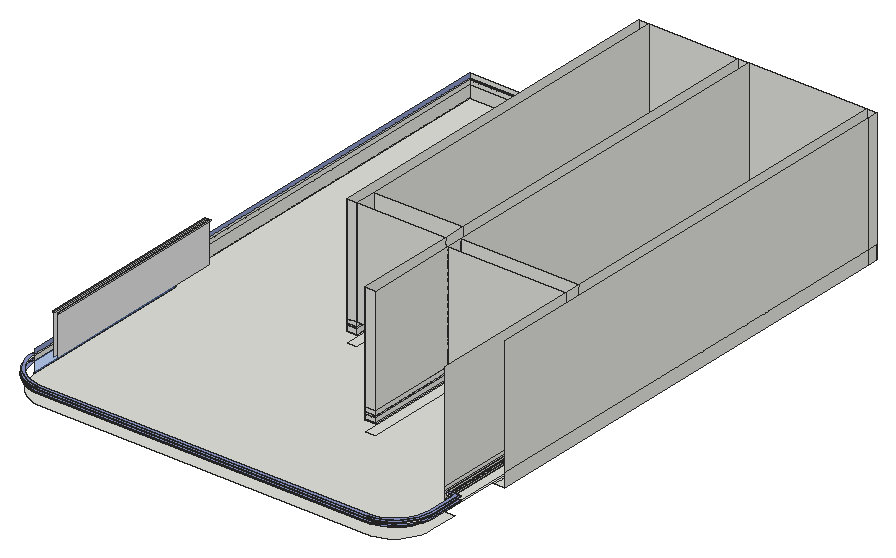
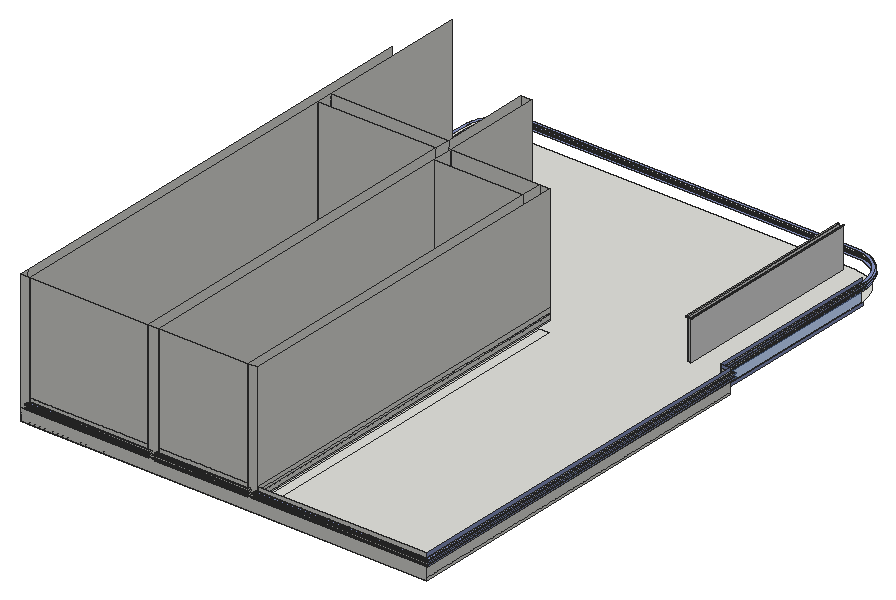
# SketchUp Ruby script. Lengths in inches.
U = 1.inch
M = Sketchup.active_model
def pt(a) = Geom::Point3d.new(a.map { |v| v * U })
def face(e, loops, mat)
  f = e.add_face(loops[0].map { |a| pt(a) })
  loops[1..].each { |l| e.add_face(l.map { |a| pt(a) }).erase! }
  f.material = f.back_material = mat if mat
  f
end
# faces: each face lists its corners as indices into pts; further lists are holes
def faces(e, pts, list, mat = nil) = list.each { |f| face(e, (f[0].is_a?(Array) ? f : [f]).map { |l| l.map { |i| pts[i] } }, mat) }
# xy, xz, yz: faces in a plane at the given z, y or x. An outline is a flat list of corners, or four numbers for a rectangle; further outlines are holes
def ring(l) = l.size == 4 ? [[l[0], l[1]], [l[2], l[1]], [l[2], l[3]], [l[0], l[3]]] : l.each_slice(2).to_a
def flat(e, list, mat, &to3) = list.each { |f| face(e, (f[0].is_a?(Array) ? f : [f]).map { |l| ring(l).map { |u, v| to3.(u, v) } }, mat) }
def xy(e, z, list, mat = nil) = flat(e, list, mat) { |x, y| [x, y, z] }
def xz(e, y, list, mat = nil) = flat(e, list, mat) { |x, z| [x, y, z] }
def yz(e, x, list, mat = nil) = flat(e, list, mat) { |y, z| [x, y, z] }
def lines(e, pts, list) = list.each { |a, b| e.add_line(pt(pts[a]), pt(pts[b])) }
# prism: a flat outline (further loops are holes) pulled along v
def prism(e, loops, v, mat = nil)
  f = face(e, loops, mat); d = Geom::Vector3d.new(v.map { |x| x * U })
  f.pushpull(f.normal.samedirection?(d) ? d.length : -d.length)
end
def box(e, o, s, mat = nil) = prism(e, [[o, [o[0] + s[0], o[1], o[2]], [o[0] + s[0], o[1] + s[1], o[2]], [o[0], o[1] + s[1], o[2]]]], [0, 0, s[2]], mat)
def at(x, y, z, deg = 0) = Geom::Transformation.translation(pt([x, y, z])) * Geom::Transformation.rotation(ORIGIN, Z_AXIS, deg.degrees)
def axes(o, x, y, z) = Geom::Transformation.new([*x, 0, *y, 0, *z, 0, *pt(o).to_a, 1])
def part(name) = M.definitions.add(name)
# library, detail: a bought-in or finely detailed component or shape, given as its bounding box
def library(name, o, s) = part(name).tap { |d| box(d.entities, o, s) }
def detail(e, o, s) = box(e.add_group.entities, o, s)
def put(e, d, t, mat = nil) = e.add_instance(d, t).tap { |i| i.material = mat if mat }
def group(e, t, mat = nil) = e.add_group.tap { |g| g.transformation = t; g.material = mat if mat }.entities
root = M.entities
M.materials.add("0326 AP 7207 CLASSIC PURPLE").color = [140, 152, 201]
M.materials.add("[Color M06]").color = [86, 86, 86]
M.materials.add("[Color M07]").color = [58, 58, 58]
M.materials.add("[Mirror 02]").color = [229, 229, 229]
M.materials.add("[Translucent Glass Blue]").color = [100, 149, 237]
M.materials["[Translucent Glass Blue]"].alpha = 0.5
xy(root,252,[[228.58,142.3125,330.09,142.75],[37.41,142.75,46.41,142.75,46.41,566.25,2.97,566.25,2.97,220.92,10.38,220.92,10.38,221.67,12.4,221.67,12.4,221.45,14.34,221.45,14.34,220.92,37.41,220.92],[46.41,142.75,181.41,557.25],[181.41,142.75,190.41,557.25],[190.41,142.75,364.41,557.25],
  [364.41,142.75,373.41,557.25],[10.38,220.92,11.125,220.92,11.125,221.45,12.4,221.45,12.4,221.67,10.38,221.67],[11.125,220.92,12.4,221.45],[12.4,220.92,14.34,221.45],[46.41,557.25,181.41,566.25],
  [181.41,557.25,190.41,566.25],[190.41,557.25,364.41,566.25],[364.41,557.25,373.41,566.25]])
xy(root,252,[[228.58,138.25,330.09,142.3125]],"[Color M07]")
xy(root,254.0625,[[45.79,26.25,340.59,26.25,344.88,26.53,349.09,27.37,353.15,28.75,357,30.65,360.57,33.03,363.8,35.86,364.41,36.56,366.625,39.09,369.01,42.66,370.91,46.51,372.29,50.57,373.125,54.78,373.41,59.0625,373.41,86.25,364.41,86.25,364.41,566.25,257.02,566.25,257.02,141.25,247.2,141.25,247.2,566.25,166.41,566.25,166.41,233.75,157.41,233.75,157.41,566.25,2.97,566.25,2.97,220.92,11.66,220.92,11.66,60.38,11.95,55.92,12.82,51.55,14.25,47.32,16.23,43.31,18.71,39.6,21.65,36.25,25.01,33.3,28.72,30.82,32.73,28.85,36.95,27.41,41.33,26.54]])
xy(root,264,[[364.41,86.25,373.41,566.25],[247.2,141.25,257.02,566.25],[157.41,233.75,166.41,566.25]])
xy(root,264.4375,[[[45.79,24.43,41.09,24.74,36.48,25.66,32.03,27.17,27.8125,29.25,23.9,31.86,20.37,34.96,17.27,38.5,14.66,42.41,12.58,46.625,11.07,51.08,10.15,55.6875,9.84,60.38,9.84,219.11,1.15,219.11,1.15,568.07,159.22,568.07,159.22,235.56,164.59,235.56,164.59,568.07,249.02,568.07,249.02,143.07,255.2,143.07,255.2,568.07,366.22,568.07,366.22,88.07,375.22,88.07,375.22,59,374.93,54.54,374.05,50.1,372.59,45.81,370.59,41.75,368.07,37.98,365.77,35.36,365.08,34.57,361.68,31.59,357.91,29.07,353.85,27.07,349.56,25.61,345.11,24.73,340.65,24.43],[45.79,26.25,340.59,26.25,344.88,26.53,349.09,27.37,353.15,28.75,357,30.65,360.57,33.03,363.8,35.86,364.41,36.56,366.625,39.09,369.01,42.66,370.91,46.51,372.29,50.57,373.125,54.78,373.41,59.0625,373.41,86.25,364.41,86.25,364.41,566.25,257.02,566.25,257.02,141.25,247.2,141.25,247.2,566.25,166.41,566.25,166.41,233.75,157.41,233.75,157.41,566.25,2.97,566.25,2.97,220.92,11.66,220.92,11.66,60.38,11.95,55.92,12.82,51.55,14.25,47.32,16.23,43.31,18.71,39.6,21.65,36.25,25.01,33.3,28.72,30.82,32.73,28.85,36.95,27.41,41.33,26.54]]],"0326 AP 7207 CLASSIC PURPLE")
xy(root,265.875,[[[45.79,23.28,40.94,23.6,36.18,24.54,31.59,26.1,27.24,28.25,23.2,30.95,19.55,34.15,16.35,37.8,13.66,41.83,11.51,46.18,9.95,50.78,9,55.54,8.6875,60.38,8.6875,217.95,0,217.95,0,569.22,160.375,569.22,160.375,236.72,163.4375,236.72,163.4375,569.22,250.17,569.22,250.17,144.22,254.05,144.22,254.05,569.22,367.375,569.22,367.375,89.22,376.375,89.22,376.375,58.97,376.08,54.39,375.16,49.8,373.66,45.37,371.59,41.17,368.99,37.28,366.64,34.6,365.9,33.76,362.38,30.67,358.49,28.07,354.29,26,349.86,24.49,345.27,23.58,340.69,23.28],[45.79,24.43,340.65,24.43,345.11,24.73,349.56,25.61,353.85,27.07,357.91,29.07,361.68,31.59,365.08,34.57,365.77,35.36,368.07,37.98,370.59,41.75,372.59,45.81,374.05,50.1,374.93,54.54,375.22,59,375.22,88.07,366.22,88.07,366.22,568.07,255.2,568.07,255.2,143.07,249.02,143.07,249.02,568.07,164.59,568.07,164.59,235.56,159.22,235.56,159.22,568.07,1.15,568.07,1.15,219.11,9.84,219.11,9.84,60.38,10.15,55.6875,11.07,51.08,12.58,46.625,14.66,42.41,17.27,38.5,20.37,34.96,23.9,31.86,27.8125,29.25,32.03,27.17,36.48,25.66,41.09,24.74]]],"0326 AP 7207 CLASSIC PURPLE")
xy(root,266.8125,[[[45.79,23.28,340.69,23.28,345.27,23.58,349.86,24.49,354.29,26,358.49,28.07,362.38,30.67,365.9,33.76,366.64,34.6,368.99,37.28,371.59,41.17,373.66,45.37,375.16,49.8,376.08,54.39,376.375,58.97,376.375,89.22,367.375,89.22,367.375,569.22,254.05,569.22,254.05,144.22,250.17,144.22,250.17,569.22,163.4375,569.22,163.4375,236.72,160.375,236.72,160.375,569.22,0,569.22,0,217.95,8.6875,217.95,8.6875,60.38,9,55.54,9.95,50.78,11.51,46.18,13.66,41.83,16.35,37.8,19.55,34.15,23.2,30.95,27.24,28.25,31.59,26.1,36.18,24.54,40.94,23.6],[45.79,24.43,41.09,24.74,36.48,25.66,32.03,27.17,27.8125,29.25,23.9,31.86,20.37,34.96,17.27,38.5,14.66,42.41,12.58,46.625,11.07,51.08,10.15,55.6875,9.84,60.38,9.84,219.11,1.15,219.11,1.15,568.07,159.22,568.07,159.22,235.56,164.59,235.56,164.59,568.07,249.02,568.07,249.02,143.07,255.2,143.07,255.2,568.07,366.22,568.07,366.22,88.07,375.22,88.07,375.22,59,374.93,54.54,374.05,50.1,372.59,45.81,370.59,41.75,368.07,37.98,365.77,35.36,365.08,34.57,361.68,31.59,357.91,29.07,353.85,27.07,349.56,25.61,345.11,24.73,340.65,24.43]]],"0326 AP 7207 CLASSIC PURPLE")
xy(root,268.875,[[[45.79,24.43,41.09,24.74,36.48,25.66,32.03,27.17,27.8125,29.25,23.9,31.86,20.37,34.96,17.27,38.5,14.66,42.41,12.58,46.625,11.07,51.08,10.15,55.6875,9.84,60.38,9.84,219.11,1.15,219.11,1.15,568.07,159.22,568.07,159.22,235.56,164.59,235.56,164.59,568.07,249.02,568.07,249.02,143.07,255.2,143.07,255.2,568.07,366.22,568.07,366.22,88.07,375.22,88.07,375.22,59,374.93,54.54,374.05,50.1,372.59,45.81,370.59,41.75,368.07,37.98,365.77,35.36,365.08,34.57,361.68,31.59,357.91,29.07,353.85,27.07,349.56,25.61,345.11,24.73,340.65,24.43],[45.79,26.25,340.59,26.25,344.88,26.53,349.09,27.37,353.15,28.75,357,30.65,360.57,33.03,363.8,35.86,364.41,36.56,366.625,39.09,369.01,42.66,370.91,46.51,372.29,50.57,373.125,54.78,373.41,59.0625,373.41,86.25,364.41,86.25,364.41,566.25,257.02,566.25,257.02,141.25,247.2,141.25,247.2,566.25,166.41,566.25,166.41,233.75,157.41,233.75,157.41,566.25,2.97,566.25,2.97,220.92,11.66,220.92,11.66,60.38,11.95,55.92,12.82,51.55,14.25,47.32,16.23,43.31,18.71,39.6,21.65,36.25,25.01,33.3,28.72,30.82,32.73,28.85,36.95,27.41,41.33,26.54]]])
xy(root,268.875,[[[45.79,23.28,40.94,23.6,36.18,24.55,31.59,26.11,27.24,28.25,23.2,30.95,19.56,34.15,16.36,37.8,13.66,41.83,11.51,46.18,9.95,50.78,9.01,55.54,8.69,60.38,8.69,217.96,0,217.96,0,569.22,160.375,569.22,160.375,236.72,163.44,236.72,163.44,569.22,250.17,569.22,250.17,144.22,254.05,144.22,254.05,569.22,367.375,569.22,367.375,89.22,376.375,89.22,376.375,58.97,376.07,54.39,375.16,49.8,373.66,45.37,371.59,41.17,368.98,37.28,366.64,34.6,365.9,33.76,362.38,30.67,358.49,28.07,354.29,26,349.86,24.5,345.27,23.58,340.69,23.28],[45.79,24.43,340.65,24.43,345.11,24.73,349.56,25.61,353.85,27.07,357.91,29.07,361.68,31.59,365.08,34.57,365.77,35.36,368.07,37.98,370.59,41.75,372.59,45.81,374.05,50.1,374.93,54.54,375.22,59,375.22,88.07,366.22,88.07,366.22,568.07,255.2,568.07,255.2,143.07,249.02,143.07,249.02,568.07,164.59,568.07,164.59,235.56,159.22,235.56,159.22,568.07,1.15,568.07,1.15,219.11,9.84,219.11,9.84,60.38,10.15,55.6875,11.07,51.08,12.58,46.625,14.66,42.41,17.27,38.5,20.37,34.96,23.9,31.86,27.8125,29.25,32.03,27.17,36.48,25.66,41.09,24.74]]],"0326 AP 7207 CLASSIC PURPLE")
xy(root,269.625,[[[45.79,23.28,340.69,23.28,345.27,23.58,349.86,24.5,354.29,26,358.49,28.07,362.38,30.67,365.9,33.76,366.64,34.6,368.98,37.28,371.59,41.17,373.66,45.37,375.16,49.8,376.07,54.39,376.375,58.97,376.375,89.22,367.375,89.22,367.375,569.22,254.05,569.22,254.05,144.22,250.17,144.22,250.17,569.22,163.44,569.22,163.44,236.72,160.375,236.72,160.375,569.22,0,569.22,0,217.96,8.69,217.96,8.69,60.38,9.01,55.54,9.95,50.78,11.51,46.18,13.66,41.83,16.36,37.8,19.56,34.15,23.2,30.95,27.24,28.25,31.59,26.11,36.18,24.55,40.94,23.6],[45.79,24.43,41.09,24.74,36.48,25.66,32.03,27.17,27.8125,29.25,23.9,31.86,20.37,34.96,17.27,38.5,14.66,42.41,12.58,46.625,11.07,51.08,10.15,55.6875,9.84,60.38,9.84,219.11,1.15,219.11,1.15,568.07,159.22,568.07,159.22,235.56,164.59,235.56,164.59,568.07,249.02,568.07,249.02,143.07,255.2,143.07,255.2,568.07,366.22,568.07,366.22,88.07,375.22,88.07,375.22,59,374.93,54.54,374.05,50.1,372.59,45.81,370.59,41.75,368.07,37.98,365.77,35.36,365.08,34.57,361.68,31.59,357.91,29.07,353.85,27.07,349.56,25.61,345.11,24.73,340.65,24.43]]],"0326 AP 7207 CLASSIC PURPLE")
xy(root,270.75,[[[45.79,24.43,340.65,24.43,345.11,24.73,349.56,25.61,353.85,27.07,357.91,29.07,361.68,31.59,365.08,34.57,365.77,35.36,368.07,37.98,370.59,41.75,372.59,45.81,374.05,50.1,374.93,54.54,375.22,59,375.22,88.07,366.22,88.07,366.22,568.07,255.2,568.07,255.2,143.07,249.02,143.07,249.02,568.07,164.59,568.07,164.59,235.56,159.22,235.56,159.22,568.07,1.15,568.07,1.15,219.11,9.84,219.11,9.84,60.38,10.15,55.6875,11.07,51.08,12.58,46.625,14.66,42.41,17.27,38.5,20.37,34.96,23.9,31.86,27.8125,29.25,32.03,27.17,36.48,25.66,41.09,24.74],[45.79,26.25,41.33,26.54,36.95,27.41,32.73,28.85,28.72,30.82,25.01,33.3,21.65,36.25,18.71,39.6,16.23,43.31,14.25,47.32,12.82,51.55,11.95,55.92,11.66,60.38,11.66,220.92,2.97,220.92,2.97,566.25,157.41,566.25,157.41,233.75,166.41,233.75,166.41,566.25,247.2,566.25,247.2,141.25,257.02,141.25,257.02,566.25,364.41,566.25,364.41,86.25,373.41,86.25,373.41,59.0625,373.125,54.78,372.29,50.57,370.91,46.51,369.01,42.66,366.625,39.09,364.41,36.56,363.8,35.86,360.57,33.03,357,30.65,353.15,28.75,349.09,27.37,344.88,26.53,340.59,26.25]]],"0326 AP 7207 CLASSIC PURPLE")
xy(root,274.4375,[[257.02,224.35,364.41,238.8],[157.41,233.75,166.41,252.68],[166.41,233.75,247.2,252.68],[257.02,238.8,364.41,566.25],[166.41,252.68,247.2,566.25]])
xz(root,141.25,[[247.2,264,257.02,264.4375],[247.2,264.4375,257.02,268.875],[247.2,268.875,257.02,270.75],[247.2,270.75,257.02,274.4375],[247.2,274.4375,257.02,372]])
xz(root,143.07,[[249.02,264.4375,255.2,265.875],[249.02,265.875,255.2,266.8125],[249.02,266.8125,255.2,268.875],[249.02,268.875,255.2,269.625],[249.02,269.625,255.2,270.75]])
xz(root,144.22,[[250.17,265.875,254.05,266.8125],[250.17,268.875,254.05,269.625]])
xz(root,217.95,[[0,265.875,8.6875,266.8125]],"0326 AP 7207 CLASSIC PURPLE")
xz(root,217.96,[[0,268.875,8.69,269.625]],"0326 AP 7207 CLASSIC PURPLE")
xz(root,219.11,[[1.15,265.875,9.84,266.8125],[1.15,268.875,9.84,269.625]])
xz(root,219.11,[[1.15,264.4375,9.84,265.875],[1.15,266.8125,9.84,268.875],[1.15,269.625,9.84,270.75]],"0326 AP 7207 CLASSIC PURPLE")
xz(root,220.92,[[2.97,252,10.38,254.0625],[10.38,252,11.125,254.0625],[11.125,252,11.66,254.0625],[12.4,252,13.8125,252.5625],[13.8125,252,15.26,252.375],
  [2.97,254.0625,11.66,264.4375],[2.97,264.4375,11.66,268.875],[2.97,268.875,11.66,270.75]])
xz(root,220.92,[[2.97,270.75,11.66,274.4375]],"0326 AP 7207 CLASSIC PURPLE")
xz(root,224.35,[[257.02,274.4375,364.41,372]])
xz(root,232.52,[[29.24,274.4375,32.41,310.4375],[29.24,310.4375,32.41,311.125]])
xz(root,233.58,[[28.18,310.4375,33.47,311.125]])
xz(root,233.75,[[157.41,264,166.41,264.4375],[157.41,264.4375,166.41,268.875],[157.41,268.875,166.41,270.75],[157.41,270.75,166.41,274.4375],[157.41,274.4375,166.41,372],
  [166.41,274.4375,247.2,372]])
xz(root,235.56,[[159.22,264.4375,164.59,265.875],[159.22,265.875,164.59,266.8125],[159.22,266.8125,164.59,268.875],[159.22,268.875,164.59,269.625],[159.22,269.625,164.59,270.75]])
xz(root,236.72,[[160.375,265.875,163.4375,266.8125],[160.375,268.875,163.44,269.625]])
xz(root,238.8,[[257.02,274.4375,364.41,372]])
xz(root,252.68,[[166.41,274.4375,247.2,372]])
xz(root,566.25,[[2.97,252,2.97,264.4375,157.41,264.4375,157.41,264,166.41,264,166.41,264.4375,247.2,264.4375,247.2,264,257.02,264,257.02,264.4375,364.41,264.4375,364.41,264,373.41,264,373.41,252],[157.41,264,166.41,372],[247.2,264,257.02,372],[364.41,264,373.41,372],[2.97,264.4375,157.41,268.875],
  [166.41,264.4375,247.2,268.875],[257.02,264.4375,364.41,268.875],[2.97,268.875,157.41,270.75],[166.41,268.875,247.2,270.75],[257.02,268.875,364.41,270.75],
  [2.97,270.75,157.41,274.4375],[166.41,270.75,247.2,274.4375],[257.02,270.75,364.41,274.4375],[166.41,274.4375,247.2,372],[257.02,274.4375,364.41,372]])
xz(root,568.07,[[1.15,264.4375,159.22,265.875],[164.59,264.4375,249.02,265.875],[255.2,264.4375,366.22,265.875],[1.15,265.875,159.22,266.8125],[164.59,265.875,249.02,266.8125],
  [255.2,265.875,366.22,266.8125],[1.15,266.8125,159.22,268.875],[164.59,266.8125,249.02,268.875],[255.2,266.8125,366.22,268.875],[1.15,268.875,159.22,269.625],
  [164.59,268.875,249.02,269.625],[255.2,268.875,366.22,269.625],[1.15,269.625,159.22,270.75],[164.59,269.625,249.02,270.75],[255.2,269.625,366.22,270.75]])
xz(root,569.22,[[0,265.875,160.375,266.8125],[163.4375,265.875,250.17,266.8125],[254.05,265.875,367.375,266.8125],[0,268.875,160.375,269.625],[163.44,268.875,250.17,269.625],
  [254.05,268.875,367.375,269.625]])
yz(root,0,[[217.95,265.875,569.22,266.8125],[217.96,268.875,569.22,269.625]],"0326 AP 7207 CLASSIC PURPLE")
yz(root,1.15,[[219.11,265.875,568.07,266.8125],[219.11,268.875,568.07,269.625]])
yz(root,1.15,[[219.11,264.4375,568.07,265.875],[219.11,266.8125,568.07,268.875],[219.11,269.625,568.07,270.75]],"0326 AP 7207 CLASSIC PURPLE")
yz(root,2.97,[[220.92,252,566.25,254.0625],[220.92,254.0625,566.25,264.4375],[220.92,264.4375,566.25,268.875],[220.92,268.875,566.25,270.75]])
yz(root,2.97,[[220.92,270.75,566.25,274.4375]],"0326 AP 7207 CLASSIC PURPLE")
yz(root,8.69,[[60.38,268.875,217.96,269.625]],"0326 AP 7207 CLASSIC PURPLE")
yz(root,9.84,[[60.38,265.875,219.11,266.8125],[60.38,268.875,219.11,269.625]])
yz(root,9.84,[[60.38,264.4375,219.11,265.875],[60.38,266.8125,219.11,268.875],[60.38,269.625,219.11,270.75]],"0326 AP 7207 CLASSIC PURPLE")
yz(root,10.38,[[60.38,252,220.92,254.0625]],"0326 AP 7207 CLASSIC PURPLE")
yz(root,11.66,[[60.38,264.4375,220.92,268.875],[60.38,268.875,220.92,270.75]])
yz(root,11.66,[[60.38,270.75,220.92,274.4375]],"0326 AP 7207 CLASSIC PURPLE")
yz(root,11.66,[[60.38,254.0625,220.92,264.4375]],"[Translucent Glass Blue]")
yz(root,12.4,[[60.38,252,220.92,252.5625]])
yz(root,13.8125,[[60.38,252,220.92,252.375],[60.38,252.375,220.92,252.5625]])
yz(root,28.18,[[60.38,310.4375,233.58,311.125]],"[Color M06]")
yz(root,29.24,[[60.38,310.4375,232.52,311.125]])
yz(root,29.24,[[60.38,274.4375,232.52,310.4375]],"[Mirror 02]")
yz(root,32.41,[[60.38,310.4375,232.52,311.125]])
yz(root,32.41,[[60.38,274.4375,232.52,310.4375]],"[Mirror 02]")
yz(root,33.47,[[60.38,310.4375,233.58,311.125]])
yz(root,157.41,[[233.75,264,566.25,264.4375],[233.75,264.4375,566.25,268.875],[233.75,268.875,566.25,270.75],[233.75,270.75,566.25,274.4375],[233.75,274.4375,566.25,372]])
yz(root,159.22,[[235.56,264.4375,568.07,265.875],[235.56,265.875,568.07,266.8125],[235.56,266.8125,568.07,268.875],[235.56,268.875,568.07,269.625],[235.56,269.625,568.07,270.75]])
yz(root,160.375,[[236.72,265.875,569.22,266.8125],[236.72,268.875,569.22,269.625]])
yz(root,163.4375,[[236.72,265.875,569.22,266.8125]])
yz(root,163.44,[[236.72,268.875,569.22,269.625]])
yz(root,164.59,[[235.56,264.4375,568.07,265.875],[235.56,265.875,568.07,266.8125],[235.56,266.8125,568.07,268.875],[235.56,268.875,568.07,269.625],[235.56,269.625,568.07,270.75]])
yz(root,166.41,[[233.75,264,566.25,264.4375],[233.75,264.4375,566.25,268.875],[233.75,268.875,566.25,270.75],[233.75,270.75,566.25,274.4375],[233.75,274.4375,252.68,372],
  [252.68,274.4375,566.25,372]])
yz(root,247.2,[[141.25,264,566.25,264.4375],[141.25,264.4375,566.25,268.875],[141.25,268.875,566.25,270.75],[141.25,270.75,566.25,274.4375],[141.25,274.4375,233.75,372],
  [233.75,274.4375,252.68,372],[252.68,274.4375,566.25,372]])
yz(root,249.02,[[143.07,264.4375,568.07,265.875],[143.07,265.875,568.07,266.8125],[143.07,266.8125,568.07,268.875],[143.07,268.875,568.07,269.625],[143.07,269.625,568.07,270.75]])
yz(root,250.17,[[144.22,265.875,569.22,266.8125],[144.22,268.875,569.22,269.625]])
yz(root,254.05,[[144.22,265.875,569.22,266.8125],[144.22,268.875,569.22,269.625]])
yz(root,255.2,[[143.07,264.4375,568.07,265.875],[143.07,265.875,568.07,266.8125],[143.07,266.8125,568.07,268.875],[143.07,268.875,568.07,269.625],[143.07,269.625,568.07,270.75]])
yz(root,257.02,[[141.25,264,566.25,264.4375],[141.25,264.4375,566.25,268.875],[141.25,268.875,566.25,270.75],[141.25,270.75,566.25,274.4375],[141.25,274.4375,224.35,372],
  [224.35,274.4375,238.8,372],[238.8,274.4375,566.25,372]])
yz(root,364.41,[[86.25,264,566.25,264.4375],[86.25,264.4375,566.25,268.875],[86.25,268.875,566.25,270.75],[86.25,270.75,566.25,274.4375],[86.25,274.4375,224.35,372],
  [224.35,274.4375,238.8,372],[238.8,274.4375,566.25,372]])
yz(root,366.22,[[88.07,264.4375,568.07,265.875],[88.07,265.875,568.07,266.8125],[88.07,266.8125,568.07,268.875],[88.07,268.875,568.07,269.625],[88.07,269.625,568.07,270.75]])
yz(root,367.375,[[89.22,265.875,569.22,266.8125],[89.22,268.875,569.22,269.625]])
yz(root,373.41,[[142.75,252,557.25,264],[557.25,252,566.25,264],[142.75,264,557.25,372],[557.25,264,566.25,372]])
